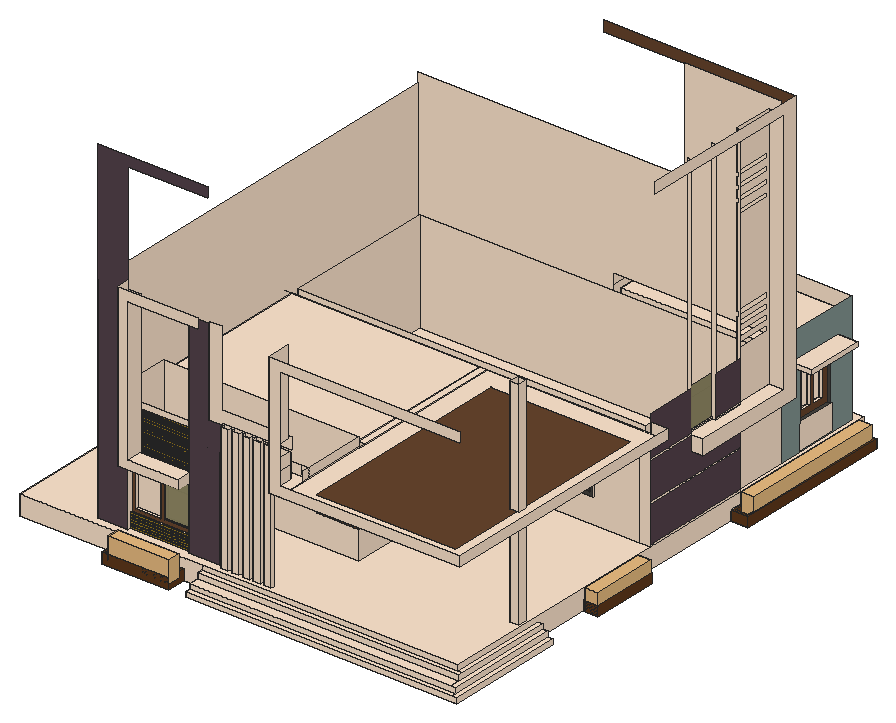
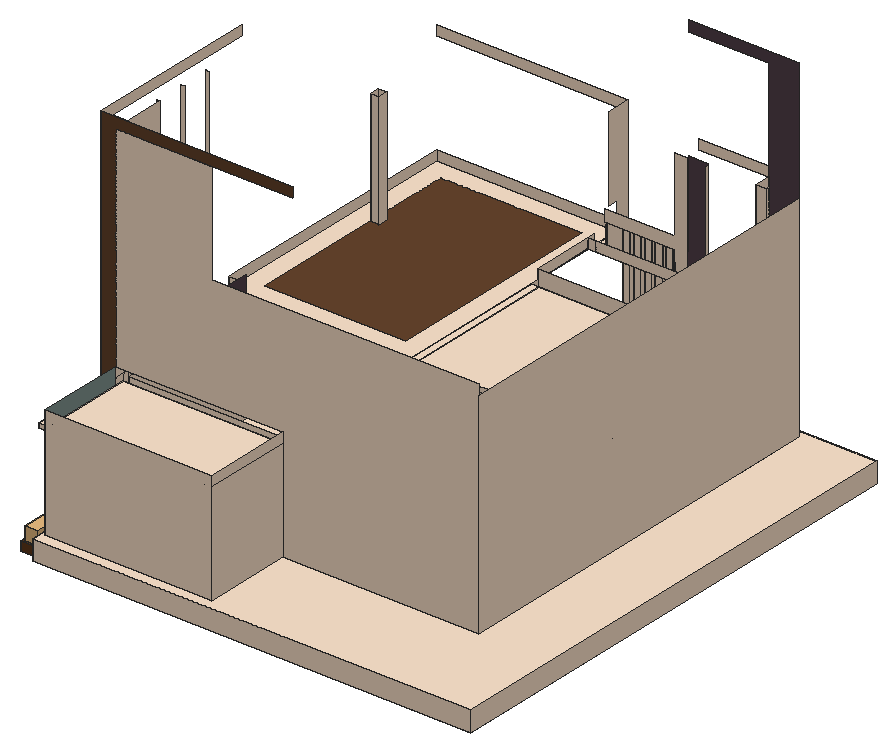
# SketchUp Ruby script. Lengths in inches.
U = 1.inch
M = Sketchup.active_model
def pt(a) = Geom::Point3d.new(a.map { |v| v * U })
def face(e, loops, mat)
  f = e.add_face(loops[0].map { |a| pt(a) })
  loops[1..].each { |l| e.add_face(l.map { |a| pt(a) }).erase! }
  f.material = f.back_material = mat if mat
  f
end
# faces: each face lists its corners as indices into pts; further lists are holes
def faces(e, pts, list, mat = nil) = list.each { |f| face(e, (f[0].is_a?(Array) ? f : [f]).map { |l| l.map { |i| pts[i] } }, mat) }
# xy, xz, yz: faces in a plane at the given z, y or x. An outline is a flat list of corners, or four numbers for a rectangle; further outlines are holes
def ring(l) = l.size == 4 ? [[l[0], l[1]], [l[2], l[1]], [l[2], l[3]], [l[0], l[3]]] : l.each_slice(2).to_a
def flat(e, list, mat, &to3) = list.each { |f| face(e, (f[0].is_a?(Array) ? f : [f]).map { |l| ring(l).map { |u, v| to3.(u, v) } }, mat) }
def xy(e, z, list, mat = nil) = flat(e, list, mat) { |x, y| [x, y, z] }
def xz(e, y, list, mat = nil) = flat(e, list, mat) { |x, z| [x, y, z] }
def yz(e, x, list, mat = nil) = flat(e, list, mat) { |y, z| [x, y, z] }
def lines(e, pts, list) = list.each { |a, b| e.add_line(pt(pts[a]), pt(pts[b])) }
# prism: a flat outline (further loops are holes) pulled along v
def prism(e, loops, v, mat = nil)
  f = face(e, loops, mat); d = Geom::Vector3d.new(v.map { |x| x * U })
  f.pushpull(f.normal.samedirection?(d) ? d.length : -d.length)
end
def box(e, o, s, mat = nil) = prism(e, [[o, [o[0] + s[0], o[1], o[2]], [o[0] + s[0], o[1] + s[1], o[2]], [o[0], o[1] + s[1], o[2]]]], [0, 0, s[2]], mat)
def at(x, y, z, deg = 0) = Geom::Transformation.translation(pt([x, y, z])) * Geom::Transformation.rotation(ORIGIN, Z_AXIS, deg.degrees)
def axes(o, x, y, z) = Geom::Transformation.new([*x, 0, *y, 0, *z, 0, *pt(o).to_a, 1])
def part(name) = M.definitions.add(name)
# library, detail: a bought-in or finely detailed component or shape, given as its bounding box
def library(name, o, s) = part(name).tap { |d| box(d.entities, o, s) }
def detail(e, o, s) = box(e.add_group.entities, o, s)
def put(e, d, t, mat = nil) = e.add_instance(d, t).tap { |i| i.material = mat if mat }
def group(e, t, mat = nil) = e.add_group.tap { |g| g.transformation = t; g.material = mat if mat }.entities
root = M.entities
M.materials.add("Brick_21_1K").color = [96, 58, 28]
M.materials.add("C01_Vanilla_Cream").color = [255, 230, 206]
M.materials.add("C04_Amber_Sunshine").color = [160, 128, 32]
M.materials.add("Carpet_04_1K").color = [85, 67, 76]
M.materials.add("Fabric_13_1K").color = [131, 150, 146]
M.materials.add("Glass_Mirror_01").color = [147, 139, 102]
M.materials["Glass_Mirror_01"].alpha = 0.98
M.materials.add("Glass_Mirror_1").color = [185, 158, 90]
M.materials.add("Wood_Floor_12_1K").color = [92, 75, 65]
M.materials.add("Wood_Planks_01_1K").color = [69, 67, 63]
M.materials.add("Wood_Veneer_15_1K").color = [107, 71, 46]
M.materials.add("Wood_Veneer_15_1K1").color = [103, 69, 45]
c1 = library("Planter with shrubs",[0,0,0],[56.02,15.3,25.28])
xy(root,-24,[[214.36,0,214.36,24,193.62,24,193.62,1.29,114.78,1.29,114.78,24,0,24,0,623.86,517,623.86,517,288.41,535,288.41,535,208.26,517,208.26,517,142.77,535,142.77,535,0],[517,427.36,537.82,616.64]],"C01_Vanilla_Cream")
xy(root,-22.75,[[520.21,430.58,534.61,613.43]],"C01_Vanilla_Cream")
xy(root,-20.26,[[519.87,211.125,532.13,285.55]],"C01_Vanilla_Cream")
xy(root,-18.25,[[117.58,4.09,190.82,21.2]],"C01_Vanilla_Cream")
xy(root,-18.03,[[529,0,535,142.77]],"C01_Vanilla_Cream")
xy(root,-18,[[214.36,0,529,6]],"C01_Vanilla_Cream")
xy(root,-13,[[[517,427.36,537.82,616.64],[520.21,430.58,534.61,613.43]]],"Brick_21_1K")
xy(root,-12.06,[[523,6,529,142.77]],"C01_Vanilla_Cream")
xy(root,-12,[[[517,208.26,535,288.41],[519.87,211.125,532.13,285.55]]],"Brick_21_1K")
xy(root,-12,[[214.36,6,523,18]],"C01_Vanilla_Cream")
xy(root,-11.23,[[[114.78,1.29,193.62,24],[117.58,4.09,190.82,21.2]]],"Brick_21_1K")
xy(root,-6.08,[[517,24,523,142.77]],"C01_Vanilla_Cream")
xy(root,0,[[[0,24,517,24,517,308.86,324,308.86,324,119.86,93,119.86,93,44.86,228,44.86,228,33.47,192,33.47,192,36.47,120,36.47,120,33.47,84,33.47,84,506.86,315,506.86,315,611.86,513,611.86,513,440.86,517,440.86,517,623.86,0,623.86],[504,118.07,514.13,128.86],[283.31,29.79,291.83,33.47],[270.62,29.79,279.14,33.47],[257.92,29.79,266.45,33.47],[245.23,29.79,253.75,33.47],[232.54,29.79,241.0625,33.47]],[84,33.47,120,33.47,120,36.47,192,36.47,192,33.47,228,33.47,228,44.86,93,44.86,93,119.86,84,119.86],[93,128.86,315,308.86],[93,317.86,504,497.86],[324,506.86,504,602.86]],"C01_Vanilla_Cream")
xy(root,6,[[342,307.36,390,308.86]],"C01_Vanilla_Cream")
xy(root,10,[[346,307.36,386,312.61],[346,312.61,386,317.86]],"Wood_Planks_01_1K")
xy(root,17.1,[[120,36.47,192,39.29]],"C01_Vanilla_Cream")
xy(root,21.1,[[124,39.29,154,42.08],[158,39.29,188,42.08],[124,42.08,154,44.86],[158,42.08,188,44.86]],"C01_Vanilla_Cream")
xy(root,30,[[414,307.36,450,308.86]],"C01_Vanilla_Cream")
xy(root,31.77,[[508.375,535.26,513,580.68]],"Wood_Planks_01_1K")
xy(root,34,[[418,307.36,430,312.61],[434,307.36,446,312.61],[418,312.61,430,317.86],[434,312.61,446,317.86]],"Wood_Planks_01_1K")
xy(root,37.47,[[315,123.86,324,173.68]],"Wood_Veneer_15_1K1")
xy(root,37.57,[[277.81,123.86,318.73,123.86,318.8125,128.86,277.81,128.86]],"C01_Vanilla_Cream")
xy(root,37.57,[[277.81,119.86,320,119.86,318.73,123.86,277.81,123.86],[318.73,123.86,324,123.86,324,128.86,318.8125,128.86]],"Wood_Veneer_15_1K1")
xy(root,38.51,[[504,542,508.375,555.97],[504,559.97,508.375,573.94]],"C01_Vanilla_Cream")
xy(root,69.79,[[124,39.29,154,42.08],[158,39.29,188,42.08],[124,42.08,154,44.86],[158,42.08,188,44.86]],"C01_Vanilla_Cream")
xy(root,73.79,[[120,18.47,192,36.47],[120,36.47,192,39.29]],"C01_Vanilla_Cream")
xy(root,75.41,[[513,368.86,517,440.86],[517,368.86,517,440.86,513,440.86,513,506.86,531,506.86,531,368.86]],"C01_Vanilla_Cream")
xy(root,81.09,[[277.81,123.86,277.81,128.86,318.8125,128.86,318.73,123.86],[315,128.86,315,173.68,319.5,173.68,318.8125,128.86]],"C01_Vanilla_Cream")
xy(root,81.09,[[277.81,119.86,320,123.86],[318.73,123.86,318.8125,128.86,324,128.86,324,123.86],[318.8125,128.86,319.5,173.68,324,173.68,324,128.86]],"Wood_Veneer_15_1K1")
xy(root,84.8125,[[132,18.47,192,36.47]],"C01_Vanilla_Cream")
xy(root,86,[[346,307.36,386,312.61],[418,307.36,430,312.61],[434,307.36,446,312.61],[346,312.61,386,317.86],[418,312.61,430,317.86],
  [434,312.61,446,317.86]],"Wood_Planks_01_1K")
xy(root,86.68,[[504,542,508.375,555.97],[504,559.97,508.375,573.94]],"C01_Vanilla_Cream")
xy(root,90,[[342,307.36,390,308.86],[414,307.36,450,308.86]],"C01_Vanilla_Cream")
xy(root,92.56,[[513,404.86,517,440.86]],"C01_Vanilla_Cream")
xy(root,93.42,[[508.375,535.26,513,580.68]],"Wood_Planks_01_1K")
xy(root,95.77,[[513,521.92,537,590.43]],"C01_Vanilla_Cream")
xy(root,100.66,[[513,521.92,537,590.43]],"C01_Vanilla_Cream")
xy(root,120,[[310.89,2.33,310.89,33.47,228,33.47,228,44.86,324,44.86,324,2.33],[[324,2.33,537,308.86],[347.11,25.4375,513.89,285.75]],[93,128.86,315,308.86],[315,128.86,324,308.86],[324,506.86,504,602.86]],"C01_Vanilla_Cream")
xy(root,120,[[347.11,25.4375,513.89,285.75]],"Wood_Veneer_15_1K1")
xz(root,0,[[214.36,-24,535,-24,535,-18.03,529,-18.03,529,-18,214.36,-18]],"C01_Vanilla_Cream")
xz(root,1.29,[[114.78,-24,193.62,-11.23]],"Brick_21_1K")
xz(root,2.33,[[310.89,120,537,120,537,132,324,132,324,252,537,252,537,264,310.89,264]],"C01_Vanilla_Cream")
xz(root,4.09,[[117.58,-18.25,190.82,-11.23]],"C01_Vanilla_Cream")
xz(root,6,[[214.36,-18,529,-18,529,-12.06,523,-12.06,523,-12,214.36,-12]],"C01_Vanilla_Cream")
xz(root,18,[[214.36,-12,523,-12,523,-6.08,214.36,-6]],"C01_Vanilla_Cream")
xz(root,18.47,[[120,73.79,192,73.79,192,84.8125,132,84.8125,132,252,213.9,252,213.9,264,120,264]],"C01_Vanilla_Cream")
xz(root,21.2,[[117.58,-18.25,190.82,-11.23]],"C01_Vanilla_Cream")
xz(root,24,[[0,-24,114.78,-24,114.78,-11.23,193.62,-11.23,193.62,-24,214.36,-24,214.36,0,0,0],[517,-6.08,517,0,214.36,0,214.36,-6]],"C01_Vanilla_Cream")
xz(root,29.79,[[232.54,0,241.0625,149.52],[245.23,0,253.75,149.52],[257.92,0,266.45,149.52],[270.62,0,279.14,149.52],[283.31,0,291.83,149.52]],"C01_Vanilla_Cream")
xz(root,33.47,[[232.54,0,241.0625,120],[245.23,0,253.75,120],[257.92,0,266.45,120],[270.62,0,279.14,120],[283.31,0,291.83,120],
  [232.54,120,241.0625,147.41],[241.0625,120,245.23,149.52],[245.23,120,253.75,147.41],[253.75,120,257.92,149.52],[257.92,120,266.45,147.41],
  [266.45,120,270.62,149.52],[270.62,120,279.14,147.41],[279.14,120,283.31,149.52],[283.31,120,291.83,147.41],[291.83,120,310.89,149.52]],"C01_Vanilla_Cream")
xz(root,33.47,[[84,0,120,0,120,384,213.9,384,213.9,396,84,396],[192,0,228,0,228,120,232.54,120,232.54,149.52,213.9,149.52,213.9,252,192,252]],"Carpet_04_1K")
xz(root,36.47,[[120,2,192,3.02],[120,5.02,192,6.04],[120,8.04,192,9.0625],[120,11.0625,192,12.08],[120,14.08,192,15.1],
  [120,73.79,192,73.79,192,84.8125,132,84.8125,132,252,120,252],[132,86.47,192,86.8125],[132,88.12,192,88.47],[132,89.77,192,90.12],[132,91.42,192,91.77],
  [132,93.07,192,93.42],[132,94.72,192,95.07],[132,96.375,192,96.72],[132,98.03,192,98.375],[132,99.68,192,100.03],
  [132,101.33,192,101.68],[132,102.98,192,103.33],[132,104.64,192,104.98],[132,106.29,192,106.64],[132,107.9375,192,108.29],
  [132,109.59,192,109.9375],[132,111.24,192,111.59],[132,112.89,192,113.24],[132,114.55,192,114.89],[132,116.2,192,116.55],
  [132,117.85,192,118.2],[132,119.5,192,119.85],[213.9,120,213.9,252,228,252,228,163.78,310.89,163.78,310.89,149.52,228,149.52,228,120],[132,121.15,192,121.5],[132,122.81,192,123.15],
  [132,124.46,192,124.81],[132,126.11,192,126.46],[132,127.76,192,128.11],[132,129.41,192,129.76]],"C01_Vanilla_Cream")
xz(root,36.47,[[120,0,192,2],[120,3.02,192,5.02],[120,6.04,192,8.04],[120,9.0625,192,11.0625],[120,12.08,192,14.08],
  [120,15.1,192,17.1],[132,84.8125,192,86.47],[132,86.8125,192,88.12],[132,88.47,192,89.77],[132,90.12,192,91.42],
  [132,91.77,192,93.07],[132,93.42,192,94.72],[132,95.07,192,96.375],[132,96.72,192,98.03],[132,98.375,192,99.68],
  [132,100.03,192,101.33],[132,101.68,192,102.98],[132,103.33,192,104.64],[132,104.98,192,106.29],[132,106.64,192,107.9375],
  [132,108.29,192,109.59],[132,109.9375,192,111.24],[132,111.59,192,112.89],[132,113.24,192,114.55],[132,114.89,192,116.2],
  [132,116.55,192,117.85],[132,118.2,192,119.5],[132,119.85,192,121.15],[132,121.5,192,122.81],[132,123.15,192,124.46],
  [132,124.81,192,126.11],[132,126.46,192,127.76],[132,128.11,192,129.41],[132,129.76,192,131.07]],"C04_Amber_Sunshine")
xz(root,39.29,[[[120,17.1,192,73.79],[124,21.1,154,69.79],[158,21.1,188,69.79]]],"Wood_Veneer_15_1K")
xz(root,42.08,[[124,21.1,154,69.79]],"C01_Vanilla_Cream")
xz(root,42.08,[[158,21.1,188,69.79]],"Glass_Mirror_01")
xz(root,44.86,[[[93,0,93,132,315,132,315,120,228,120,228,0],[124,21.1,154,69.79],[158,21.1,188,69.79]],[315,120,324,132]],"C01_Vanilla_Cream")
xz(root,118.07,[[504,0,514.13,254.95]],"C01_Vanilla_Cream")
xz(root,119.86,[[93,0,324,0,324,33.57,273.81,33.57,273.81,85.09,324,85.09,324,132,93,132]],"C01_Vanilla_Cream")
xz(root,119.86,[[[273.81,33.57,324,85.09],[277.81,37.57,320,81.09]]],"Wood_Veneer_15_1K1")
xz(root,123.86,[[315,37.47,324,37.57],[277.81,37.57,318.73,81.09],[318.73,37.57,318.73,81.09,320,81.09]],"C01_Vanilla_Cream")
xz(root,123.86,[[318.73,37.57,320,81.09,324,81.09,324,37.57]],"Wood_Veneer_15_1K1")
xz(root,128.86,[[93,0,93,120,315,120,315,81.09,277.81,81.09,277.81,37.57,315,37.57,315,0],[504,0,514.13,254.95]],"C01_Vanilla_Cream")
xz(root,142.77,[[517,-24,535,-18.03],[517,-18.03,529,-12.06],[517,-12.06,523,-6.08]],"C01_Vanilla_Cream")
xz(root,173.68,[[315,37.47,324,81.09]],"Wood_Veneer_15_1K1")
xz(root,208.26,[[517,-24,535,-12]],"Brick_21_1K")
xz(root,211.125,[[519.87,-20.26,532.13,-12]],"C01_Vanilla_Cream")
xz(root,285.55,[[519.87,-20.26,532.13,-12]],"C01_Vanilla_Cream")
xz(root,288.41,[[517,-24,535,-12]],"Brick_21_1K")
xz(root,307.36,[[[342,6,390,90],[346,10,386,86]],[[414,30,450,90],[418,34,430,86],[434,34,446,86]]],"Wood_Planks_01_1K")
xz(root,308.86,[[93,0,315,120],[[324,0,504,120],[342,6,390,90],[414,30,450,90]],[504,0,517,120],[517,120,537,131.96]],"C01_Vanilla_Cream")
xz(root,312.61,[[418,34,430,86],[434,34,446,86]],"Glass_Mirror_01")
xz(root,312.61,[[346,10,386,86]],"Wood_Floor_12_1K")
xz(root,317.86,[[[93,0,504,120],[346,10,386,86],[418,34,430,86],[434,34,446,86]]],"C01_Vanilla_Cream")
xz(root,368.86,[[513,75.41,517,92.56],[517,75.41,531,75.41,531,92.66,517,92.58],[513,92.56,513,384,517,384,517,92.58],[513,92.56,517,92.56,517,92.57,515,92.57],[515,92.57,517,92.57,517,92.58]],"C01_Vanilla_Cream")
xz(root,404.86,[[513,92.56,517,384]],"C01_Vanilla_Cream")
xz(root,427.36,[[517,-24,537.82,-13]],"Brick_21_1K")
xz(root,430.58,[[520.21,-22.75,534.61,-13]],"Brick_21_1K")
xz(root,440.86,[[513,0,517,75.41],[513,92.56,513,184.72,516,184.72,516,190.64,513,190.64,513,304.79,516,304.79,516,310.71,513,310.71,513,318.59,516,318.59,516,324.51,513,324.51,513,332.38,516,332.38,516,338.3,513,338.3,513,384,517,384,517,92.56]],"C01_Vanilla_Cream")
xz(root,488.83,[[513,92.56,531,92.66,531,384,513,384]],"C01_Vanilla_Cream")
xz(root,497.86,[[93,0,504,120]],"C01_Vanilla_Cream")
xz(root,506.86,[[84,0,84,264,399,264,399,384,513,384,513,132,315,132,315,0],[324,0,504,120]],"C01_Vanilla_Cream")
xz(root,506.86,[[513,75.41,513,384,303.34,384,303.34,396,531,396,531,75.41]],"Wood_Veneer_15_1K1")
xz(root,521.92,[[513,95.77,537,100.66]],"C01_Vanilla_Cream")
xz(root,535.26,[[508.375,31.77,513,93.42]],"Wood_Planks_01_1K")
xz(root,542,[[504,38.51,508.375,86.68]],"C01_Vanilla_Cream")
xz(root,555.97,[[504,38.51,508.375,86.68]],"C01_Vanilla_Cream")
xz(root,559.97,[[504,38.51,508.375,86.68]],"C01_Vanilla_Cream")
xz(root,573.94,[[504,38.51,508.375,86.68]],"C01_Vanilla_Cream")
xz(root,580.68,[[508.375,31.77,513,93.42]],"Wood_Planks_01_1K")
xz(root,590.43,[[513,95.77,537,100.66]],"C01_Vanilla_Cream")
xz(root,602.86,[[324,0,504,120]],"C01_Vanilla_Cream")
xz(root,611.86,[[315,0,513,132]],"C01_Vanilla_Cream")
xz(root,613.43,[[520.21,-22.75,534.61,-13]],"Brick_21_1K")
xz(root,616.64,[[517,-24,537.82,-13]],"Brick_21_1K")
xz(root,623.86,[[0,-24,517,0]],"C01_Vanilla_Cream")
yz(root,0,[[24,-24,623.86,0]],"C01_Vanilla_Cream")
yz(root,84,[[33.47,0,506.86,252]],"C01_Vanilla_Cream")
yz(root,93,[[44.86,0,119.86,132],[128.86,0,308.86,120],[317.86,0,497.86,120]],"C01_Vanilla_Cream")
yz(root,114.78,[[1.29,-24,24,-11.23]],"Brick_21_1K")
yz(root,117.58,[[4.09,-18.25,21.2,-11.23]],"C01_Vanilla_Cream")
yz(root,120,[[33.47,0,36.47,0,36.47,17.1,39.29,17.1,39.29,73.79,33.47,73.79],[18.47,73.79,33.47,264],[33.47,73.79,36.47,252]],"C01_Vanilla_Cream")
yz(root,124,[[39.29,21.1,42.08,69.79],[42.08,21.1,44.86,69.79]],"C01_Vanilla_Cream")
yz(root,132,[[18.47,84.8125,36.47,252]],"C01_Vanilla_Cream")
yz(root,154,[[39.29,21.1,42.08,69.79],[42.08,21.1,44.86,69.79]],"C01_Vanilla_Cream")
yz(root,158,[[39.29,21.1,42.08,69.79],[42.08,21.1,44.86,69.79]],"C01_Vanilla_Cream")
yz(root,188,[[39.29,21.1,42.08,69.79],[42.08,21.1,44.86,69.79]],"C01_Vanilla_Cream")
yz(root,190.82,[[4.09,-18.25,21.2,-11.23]],"C01_Vanilla_Cream")
yz(root,192,[[33.47,0,33.47,73.79,39.29,73.79,39.29,17.1,36.47,17.1,36.47,0],[18.47,73.79,33.47,84.8125],[33.47,73.79,36.47,84.8125],[33.47,84.8125,36.47,249.4]],"C01_Vanilla_Cream")
yz(root,193.62,[[1.29,-24,24,-11.23]],"Brick_21_1K")
yz(root,214.36,[[0,-24,24,-18],[6,-18,24,-12],[18,-12,24,-6]],"C01_Vanilla_Cream")
yz(root,228,[[33.47,0,36.13,120],[36.47,0,44.86,120],[36.13,120,36.47,135.59]],"C01_Vanilla_Cream")
yz(root,232.54,[[29.79,0,33.47,149.52]],"C01_Vanilla_Cream")
yz(root,241.0625,[[29.79,0,33.47,149.52]],"C01_Vanilla_Cream")
yz(root,245.23,[[29.79,0,33.47,149.52]],"C01_Vanilla_Cream")
yz(root,253.75,[[29.79,0,33.47,149.52]],"C01_Vanilla_Cream")
yz(root,257.92,[[29.79,0,33.47,149.52]],"C01_Vanilla_Cream")
yz(root,266.45,[[29.79,0,33.47,149.52]],"C01_Vanilla_Cream")
yz(root,270.62,[[29.79,0,33.47,149.52]],"C01_Vanilla_Cream")
yz(root,277.81,[[123.86,37.57,128.86,81.09]],"C01_Vanilla_Cream")
yz(root,277.81,[[119.86,37.57,123.86,81.09]],"Wood_Veneer_15_1K1")
yz(root,279.14,[[29.79,0,33.47,149.52]],"C01_Vanilla_Cream")
yz(root,283.31,[[29.79,0,33.47,149.52]],"C01_Vanilla_Cream")
yz(root,291.83,[[29.79,0,33.47,149.52]],"C01_Vanilla_Cream")
yz(root,310.89,[[2.33,120,2.33,264,30.68,264,30.68,163.78,18.47,163.78,18.47,149.52,33.47,149.52,33.47,135.59,18.47,135.59,18.47,120],[18.47,120,33.47,135.59]],"C01_Vanilla_Cream")
yz(root,315,[[128.86,0,128.86,37.47,173.68,37.47,173.68,81.09,128.86,81.09,128.86,120,308.86,120,308.86,0],[506.86,0,611.86,120],[506.86,120,611.86,132]],"C01_Vanilla_Cream")
yz(root,320,[[119.86,37.57,119.86,81.09,123.86,81.09]],"Wood_Veneer_15_1K1")
yz(root,324,[[119.86,0,308.86,0,308.86,120,119.86,120,119.86,85.09,177.68,85.09,177.68,33.47,119.86,33.47],[506.86,0,602.86,120],[36.47,120,44.86,120.82],[44.86,120,119.86,120.82],[36.47,120.82,44.86,132],
  [44.86,120.82,119.86,132]],"C01_Vanilla_Cream")
yz(root,324,[[[119.86,33.47,177.68,85.09],[123.86,37.47,173.68,81.09]]],"Wood_Veneer_15_1K1")
yz(root,342,[[307.36,6,308.86,90]],"C01_Vanilla_Cream")
yz(root,346,[[307.36,10,312.61,86],[312.61,10,317.86,86]],"Wood_Planks_01_1K")
yz(root,386,[[307.36,10,312.61,86],[312.61,10,317.86,86]],"Wood_Planks_01_1K")
yz(root,390,[[307.36,6,308.86,90]],"C01_Vanilla_Cream")
yz(root,414,[[307.36,30,308.86,90]],"C01_Vanilla_Cream")
yz(root,418,[[307.36,34,312.61,86],[312.61,34,317.86,86]],"Wood_Planks_01_1K")
yz(root,430,[[307.36,34,312.61,86],[312.61,34,317.86,86]],"Wood_Planks_01_1K")
yz(root,434,[[307.36,34,312.61,86],[312.61,34,317.86,86]],"Wood_Planks_01_1K")
yz(root,446,[[307.36,34,312.61,86],[312.61,34,317.86,86]],"Wood_Planks_01_1K")
yz(root,450,[[307.36,30,308.86,90]],"C01_Vanilla_Cream")
yz(root,504,[[118.07,0,128.86,254.95],[317.86,0,497.86,120],[[506.86,0,602.86,120],[559.97,38.51,573.94,86.68],[542,38.51,555.97,86.68]]],"C01_Vanilla_Cream")
yz(root,508.375,[[[535.26,31.77,580.68,93.42],[559.97,38.51,573.94,86.68],[542,38.51,555.97,86.68]]],"Wood_Veneer_15_1K1")
yz(root,513,[[440.86,0,506.86,75.41],[535.26,1.4375,581.66,31.77],[368.86,75.41,494.76,75.41,494.76,120,488.83,120,488.83,92.56,368.86,92.56],[494.76,75.41,506.86,120],[368.86,92.56,404.86,94.56],
  [[440.86,92.56,488.83,92.56,488.83,384,440.86,384,440.86,338.3,486.47,338.3,486.47,332.38,440.86,332.38,440.86,324.51,486.47,324.51,486.47,318.59,440.86,318.59,440.86,310.71,486.47,310.71,486.47,304.79,440.86,304.79,440.86,190.64,486.47,190.64,486.47,184.72,440.86,184.72],[440.92,173.03,486.47,178.95],[440.92,161.34,486.47,167.26],[440.92,149.65,486.47,155.57],[441.08,290.99,486.47,296.91]],[488.83,120,494.76,132],[494.76,120,506.86,132]],"C01_Vanilla_Cream")
yz(root,513,[[[506.86,0,611.86,132],[535.26,1.4375,535.26,93.42,580.68,93.42,580.68,31.77,581.66,31.77,581.66,1.4375],[521.92,95.77,590.43,100.66]]],"Fabric_13_1K")
yz(root,513,[[368.86,94.56,404.86,140.8]],"Glass_Mirror_01")
yz(root,514.13,[[118.07,0,128.86,254.95]],"C01_Vanilla_Cream")
yz(root,517,[[142.77,-24,208.26,-24,208.26,-12,288.41,-12,288.41,-24,427.36,-24,427.36,-13,616.64,-13,616.64,-24,623.86,-24,623.86,0,24,0,24,-6.08,142.77,-6.08],[427.36,-24,616.64,-13],[308.86,0,440.86,2],[308.86,45.51,440.86,47.51],[308.86,91.68,368.86,93.68],
  [404.86,92.56,440.86,93.02],[404.86,93.02,440.86,95.02]],"C01_Vanilla_Cream")
yz(root,517,[[308.86,2,440.86,45.51],[308.86,47.51,440.86,47.51,440.86,75.41,368.86,75.41,368.86,91.68,308.86,91.68],[308.86,93.68,368.86,141.18],[404.86,95.02,440.86,141.18]],"Carpet_04_1K")
yz(root,519.87,[[211.125,-20.26,285.55,-12]],"C01_Vanilla_Cream")
yz(root,520.21,[[430.58,-22.75,613.43,-13]],"Brick_21_1K")
yz(root,523,[[6,-12.06,142.77,-12.06,142.77,-6.08,18,-6.08,18,-12,6,-12]],"C01_Vanilla_Cream")
yz(root,529,[[0,-18.03,142.77,-18.03,142.77,-12.06,6,-12.06,6,-18,0,-18]],"C01_Vanilla_Cream")
yz(root,531,[[368.86,75.41,506.86,75.41,506.86,396,297.92,396,297.92,384,488.83,384,488.83,92.66,368.86,92.66]],"C01_Vanilla_Cream")
yz(root,532.13,[[211.125,-20.26,285.55,-12]],"C01_Vanilla_Cream")
yz(root,534.61,[[430.58,-22.75,613.43,-13]],"C01_Vanilla_Cream")
yz(root,535,[[208.26,-24,288.41,-12]],"Brick_21_1K")
yz(root,535,[[0,-24,142.77,-18.03]],"C01_Vanilla_Cream")
yz(root,537,[[521.92,95.77,590.43,100.66],[2.33,120,308.86,120,308.86,131.96,298.66,131.96,298.66,132,2.33,132]],"C01_Vanilla_Cream")
yz(root,537.82,[[427.36,-24,616.64,-13]],"Brick_21_1K")
p = [[517,24,-6.08],[214.36,24,-6],[214.36,18,-6],[523,18,-6.08],[523,24,-6.08],[318.73,123.86,37.57],
  [320,119.86,37.57],[320,123.86,81.09],[318.8125,128.86,37.57],[319.5,173.68,37.57],[319.5,173.68,81.09],[318.8125,128.86,81.09],
  [318.73,123.86,81.09],[531,488.83,92.66],[513,488.83,92.56],[513,440.86,92.56],[513,404.86,92.56],[513,368.86,92.56],
  [515,368.86,92.57],[517,368.86,92.58],[531,368.86,92.66],[324,36.47,120.82],[324,2.33,120.82],[213.9,36.47,120],
  [213.9,33.47,120],[310.89,36.47,147.41],[310.89,36.47,120],[84,308.86,120],[93,308.86,120],[324,602.86,120],
  [324,611.86,120],[504,602.86,120],[504,611.86,120]]
faces(root,p,[[0,1,2,3,4],[13,14,15,16,17,18,19,20]],"C01_Vanilla_Cream")
faces(root,p,[[5,6,7]],"Wood_Veneer_15_1K1")
faces(root,p,[[5,8,9,10,11,12]],"Glass_Mirror_1")
lines(root,p,[[21,22],[23,24],[25,26],[27,28],[29,30],[31,32]])
put(root,c1,axes([535,208.26,-23],[0,1.40353,0],[-1,0,0],[0,0,1]),"C01_Vanilla_Cream")
put(root,c1,axes([535,438.45,-23],[0,3.12377,0],[-1,0,0],[0,0,1]),"C01_Vanilla_Cream")
put(root,c1,axes([121.77,1.29,-17.73],[1.28264,0,0],[0,1,0],[0,0,1]),"C01_Vanilla_Cream")
